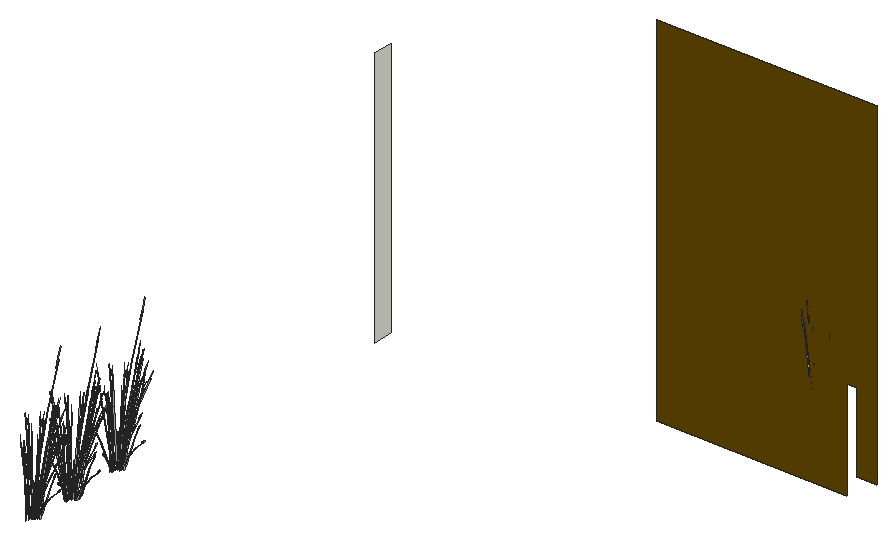
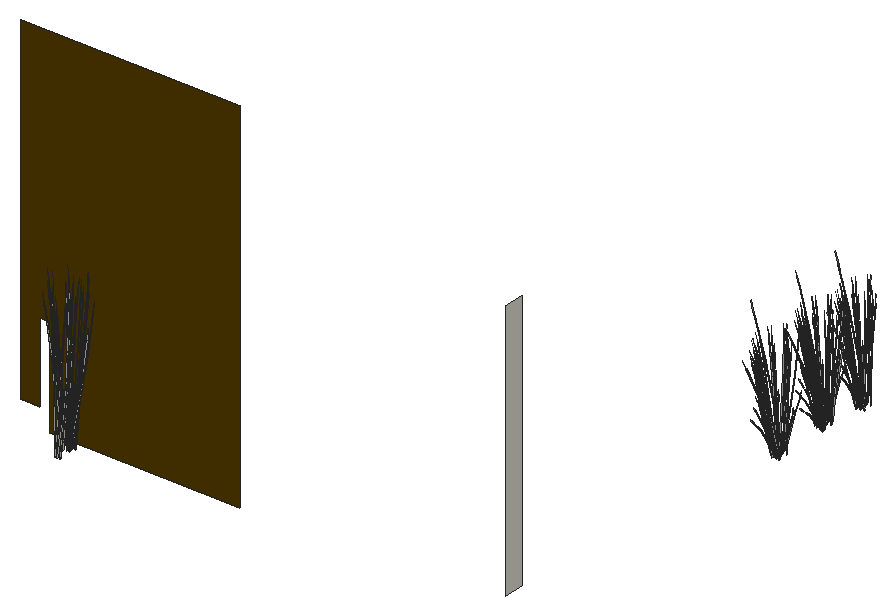
# SketchUp Ruby script. Lengths in inches.
U = 1.inch
M = Sketchup.active_model
def pt(a) = Geom::Point3d.new(a.map { |v| v * U })
def face(e, loops, mat)
  f = e.add_face(loops[0].map { |a| pt(a) })
  loops[1..].each { |l| e.add_face(l.map { |a| pt(a) }).erase! }
  f.material = f.back_material = mat if mat
  f
end
# faces: each face lists its corners as indices into pts; further lists are holes
def faces(e, pts, list, mat = nil) = list.each { |f| face(e, (f[0].is_a?(Array) ? f : [f]).map { |l| l.map { |i| pts[i] } }, mat) }
# xy, xz, yz: faces in a plane at the given z, y or x. An outline is a flat list of corners, or four numbers for a rectangle; further outlines are holes
def ring(l) = l.size == 4 ? [[l[0], l[1]], [l[2], l[1]], [l[2], l[3]], [l[0], l[3]]] : l.each_slice(2).to_a
def flat(e, list, mat, &to3) = list.each { |f| face(e, (f[0].is_a?(Array) ? f : [f]).map { |l| ring(l).map { |u, v| to3.(u, v) } }, mat) }
def xy(e, z, list, mat = nil) = flat(e, list, mat) { |x, y| [x, y, z] }
def xz(e, y, list, mat = nil) = flat(e, list, mat) { |x, z| [x, y, z] }
def yz(e, x, list, mat = nil) = flat(e, list, mat) { |y, z| [x, y, z] }
def lines(e, pts, list) = list.each { |a, b| e.add_line(pt(pts[a]), pt(pts[b])) }
# prism: a flat outline (further loops are holes) pulled along v
def prism(e, loops, v, mat = nil)
  f = face(e, loops, mat); d = Geom::Vector3d.new(v.map { |x| x * U })
  f.pushpull(f.normal.samedirection?(d) ? d.length : -d.length)
end
def box(e, o, s, mat = nil) = prism(e, [[o, [o[0] + s[0], o[1], o[2]], [o[0] + s[0], o[1] + s[1], o[2]], [o[0], o[1] + s[1], o[2]]]], [0, 0, s[2]], mat)
def at(x, y, z, deg = 0) = Geom::Transformation.translation(pt([x, y, z])) * Geom::Transformation.rotation(ORIGIN, Z_AXIS, deg.degrees)
def axes(o, x, y, z) = Geom::Transformation.new([*x, 0, *y, 0, *z, 0, *pt(o).to_a, 1])
def part(name) = M.definitions.add(name)
# library, detail: a bought-in or finely detailed component or shape, given as its bounding box
def library(name, o, s) = part(name).tap { |d| box(d.entities, o, s) }
def detail(e, o, s) = box(e.add_group.entities, o, s)
def put(e, d, t, mat = nil) = e.add_instance(d, t).tap { |i| i.material = mat if mat }
def group(e, t, mat = nil) = e.add_group.tap { |g| g.transformation = t; g.material = mat if mat }.entities
root = M.entities
M.materials.add("D01_Frost_White").color = [238, 238, 227]
M.materials.add("D08_Bronzed_Mustard").color = [102, 74, 0]
M.materials.add("LightPink_Translucent").color = [144, 107, 117]
M.materials["LightPink_Translucent"].alpha = 0.75
c1 = part("blade")
p = [[2.15,0.21,22],[0,0.17,0],[0.09,0.45,0],[2.18,0.31,22],[2.29,0.31,22],[0.38,0.45,0],
  [2.48,0.24,33],[2.49,0.24,33],[2.48,0.22,33]]
faces(c1.entities,p,[[0,1,2,3],[4,5,2,3],[6,3,4,7],[8,0,3,6]])
c2 = part("seeds")
p = [[0.3,-0.1,1.38],[-0.01,-0.03,1.59],[-0.01,-0.03,0.03],[0.14,-0.07,-0.07],[0.29,-0.03,3],[0.15,0.01,3.11]]
faces(c2.entities,p,[[0,1,2,3],[1,0,4,5]],"LightPink_Translucent")
c3 = part("blade with seeds")
put(c3.entities,c1,at(0,0,0))
put(c3.entities,c2,axes([2.4,0.25,30.99],[1.5799,-0.05474,1.17369],[-0.12525,1.92788,0.29478],[-0.07173,-0.02425,1.56792]))
xz(root,373,[[382,150,382,258,448,258,448,156,442,156,442,180,439,180,439,150]],"D08_Bronzed_Mustard")
yz(root,307,[[361,150,367,228]],"D01_Frost_White")
put(root,c3,axes([297.88,255.65,151],[0.30197,-0.1603,0.05432],[0.1478,0.29231,0.42765],[-0.02916,-0.12885,0.65209]))
put(root,c3,axes([296.1,245.72,150.27],[-0.09368,-0.15143,1.44779],[0.43286,-0.12749,0.11706],[0.09783,0.23774,0.61892]))
put(root,c3,axes([296.9,260.5,150.98],[0.05195,0.07595,1.47793],[0.41921,0.02984,-0.23373],[0.04216,0.1675,0.11853]))
put(root,c3,axes([296.28,277.23,151.25],[0.40102,-0.2196,-0.10273],[0.19707,0.38974,-0.57019],[0.05291,0.16424,0.8664]))
put(root,c3,axes([297.78,255.68,151],[0.4038,0.12331,0.40553],[-0.13808,0.40538,0.33437],[-0.02427,-0.15942,0.83914]))
put(root,c3,axes([298.33,272.88,150.98],[-0.04162,0.03603,1.49853],[-0.40776,-0.12155,-0.1416],[-0.01476,-0.15722,0.26519]))
put(root,c3,axes([298.01,273.92,151.25],[-0.45039,-0.02337,-0.10273],[0.01231,-0.44247,-0.57019],[0.03129,-0.17041,0.8664]))
put(root,c3,axes([297.12,259.47,151.27],[0.12355,-0.36271,0.29918],[0.36044,0.10579,-0.38624],[0.03305,0.14603,0.73904]))
put(root,c3,axes([296.51,246.37,151.27],[-0.06329,-0.37991,0.29918],[0.36182,-0.10032,-0.38624],[0.09718,0.10887,0.73904]))
put(root,c3,axes([296.75,244.18,150.78],[-0.35411,-0.24507,1.16821],[0.37391,-0.38156,0.50405],[0.11425,0.22994,1.12919]))
put(root,c3,axes([297.22,242.98,150.82],[0.27728,-0.24833,-0.29918],[0.26248,0.28355,0.38624],[0.03994,-0.14407,0.73904]))
put(root,c3,axes([296.16,246.9,150.98],[0.00121,-0.0571,1.49853],[0.35119,-0.25193,-0.1416],[0.12199,0.08992,0.26519]))
put(root,c3,axes([297.33,243.11,151],[0.33677,0.02198,0.05432],[-0.00923,0.33185,0.42765],[0.03524,-0.12712,0.65209]))
put(root,c3,axes([297.4,277.28,151],[-0.4076,0.10824,0.40553],[-0.07074,-0.4246,0.33437],[0.09586,0.12514,0.83914]))
put(root,c3,axes([297.22,243.08,151],[0.29182,0.32181,0.40553],[-0.3099,0.27755,0.33437],[0.05383,-0.15098,0.83914]))
put(root,c3,axes([297.32,277.37,151],[-0.18625,0.29962,0.05432],[-0.26523,-0.17444,0.42765],[0.08575,0.09606,0.65209]))
put(root,c3,axes([297,259.63,151.25],[0.40102,-0.2196,-0.10273],[0.19707,0.38974,-0.57019],[0.05291,0.16424,0.8664]))
put(root,c3,axes([296.85,276.38,150.27],[-0.09368,-0.15143,1.44779],[0.43286,-0.12749,0.11706],[0.09783,0.23774,0.61892]))
put(root,c3,axes([299.04,255.28,150.98],[-0.04162,0.03603,1.49853],[-0.40776,-0.12155,-0.1416],[-0.01476,-0.15722,0.26519]))
put(root,c3,axes([298.72,256.32,151.25],[-0.45039,-0.02337,-0.10273],[0.01231,-0.44247,-0.57019],[0.03129,-0.17041,0.8664]))
put(root,c3,axes([298.55,256.38,151.27],[-0.27728,0.24833,0.29918],[-0.26248,-0.28355,-0.38624],[0.03994,-0.14407,0.73904]))
put(root,c3,axes([297.56,244.1,151.27],[-0.35672,0.06741,0.29918],[-0.09419,-0.38534,-0.38624],[0.10222,-0.1035,0.73904]))
put(root,c3,axes([296.53,243.03,150.27],[-0.0763,0.16212,1.44779],[-0.3201,-0.3355,0.11706],[0.1444,-0.2091,0.61892]))
put(root,c3,axes([296.48,246.5625,151.25],[0.2442,-0.40372,-0.10273],[0.35364,0.23259,-0.57019],[0.12293,0.11406,0.8664]))
put(root,c3,axes([297.51,274.84,150.78],[-0.35411,-0.24507,1.16821],[0.37391,-0.38156,0.50405],[0.11425,0.22994,1.12919]))
put(root,c3,axes([297.98,273.64,150.82],[0.27728,-0.24833,-0.29918],[0.26248,0.28355,0.38624],[0.03994,-0.14407,0.73904]))
put(root,c3,axes([297.74,244.14,151.25],[-0.37908,-0.26007,-0.10273],[0.21839,-0.37663,-0.57019],[0.1071,-0.13092,0.8664]))
put(root,c3,axes([296.91,277.55,150.98],[0.00121,-0.0571,1.49853],[0.35119,-0.25193,-0.1416],[0.12199,0.08992,0.26519]))
put(root,c3,axes([298.08,273.77,151],[0.33677,0.02198,0.05432],[-0.00923,0.33185,0.42765],[0.03524,-0.12712,0.65209]))
put(root,c3,axes([298.12,259.68,151],[-0.4076,0.10824,0.40553],[-0.07074,-0.4246,0.33437],[0.09586,0.12514,0.83914]))
put(root,c3,axes([298.04,259.76,151],[-0.18625,0.29962,0.05432],[-0.26523,-0.17444,0.42765],[0.08575,0.09606,0.65209]))
put(root,c3,axes([298.42,273.22,150.98],[-0.00396,-0.09387,1.47793],[-0.33411,-0.2713,-0.23373],[0.05166,-0.16446,0.11853]))
put(root,c3,axes([297.57,258.77,150.27],[-0.09368,-0.15143,1.44779],[0.43286,-0.12749,0.11706],[0.09783,0.23774,0.61892]))
put(root,c3,axes([297.98,273.74,151],[0.29182,0.32181,0.40553],[-0.3099,0.27755,0.33437],[0.05383,-0.15098,0.83914]))
put(root,c3,axes([297.23,245.85,151.27],[-0.23317,-0.29531,0.29918],[0.26625,-0.27955,-0.38624],[0.13527,0.04253,0.73904]))
put(root,c3,axes([297.44,246.12,151],[-0.02064,0.35866,0.05432],[-0.3116,-0.00983,0.42765],[0.11936,0.03753,0.65209]))
put(root,c3,axes([297.47,246.01,151],[-0.30217,0.31079,0.40553],[-0.2606,-0.33005,0.33437],[0.14177,0.05733,0.83914]))
put(root,c3,axes([298.25,246.05,150.32],[-0.07843,-0.39649,-0.0295],[0.37072,-0.09115,-0.13375],[0.07742,0.02514,0.44114]))
put(root,c3,axes([297.61,245.03,151.27],[-0.34057,-0.13158,0.29918],[0.09933,-0.38387,-0.38624],[0.13712,-0.0352,0.73904]))
put(root,c3,axes([297.98,259.41,151.27],[-0.06329,-0.37991,0.29918],[0.36182,-0.10032,-0.38624],[0.09718,0.10887,0.73904]))
put(root,c3,axes([297.29,273.68,150.27],[-0.0763,0.16212,1.44779],[-0.3201,-0.3355,0.11706],[0.1444,-0.2091,0.61892]))
put(root,c3,axes([298.23,257.23,150.78],[-0.35411,-0.24507,1.16821],[0.37391,-0.38156,0.50405],[0.11425,0.22994,1.12919]))
put(root,c3,axes([297.88,244.04,151],[0.28133,0.19836,0.05432],[-0.16379,0.28248,0.42765],[0.0902,-0.09132,0.65209]))
put(root,c3,axes([297.23,277.22,151.25],[0.2442,-0.40372,-0.10273],[0.35364,0.23259,-0.57019],[0.12293,0.11406,0.8664]))
put(root,c3,axes([297.63,259.95,150.98],[0.00121,-0.0571,1.49853],[0.35119,-0.25193,-0.1416],[0.12199,0.08992,0.26519]))
put(root,c3,axes([298.8,256.16,151],[0.33677,0.02198,0.05432],[-0.00923,0.33185,0.42765],[0.03524,-0.12712,0.65209]))
put(root,c3,axes([298.5,274.79,151.25],[-0.37908,-0.26007,-0.10273],[0.21839,-0.37663,-0.57019],[0.1071,-0.13092,0.8664]))
put(root,c3,axes([297.8,243.96,151],[0.10163,0.43409,0.40553],[-0.39868,0.07534,0.33437],[0.1175,-0.10209,0.83914]))
put(root,c3,axes([299.13,255.61,150.98],[-0.00396,-0.09387,1.47793],[-0.33411,-0.2713,-0.23373],[0.05166,-0.16446,0.11853]))
put(root,c3,axes([298.69,256.13,151],[0.29182,0.32181,0.40553],[-0.3099,0.27755,0.33437],[0.05383,-0.15098,0.83914]))
put(root,c3,axes([296.72,245.25,150.27],[-0.15222,-0.08126,1.44779],[0.31502,-0.34091,0.11706],[0.19634,0.15379,0.61892]))
put(root,c3,axes([298.67,244.03,150.98],[-0.05353,-0.00358,1.49853],[-0.22227,-0.38383,-0.1416],[0.08926,-0.1262,0.26519]))
put(root,c3,axes([297.85,243.875,150.82],[0.35672,-0.06741,-0.29918],[0.09419,0.38534,0.38624],[0.10222,-0.1035,0.73904]))
put(root,c3,axes([298.2,276.78,151],[-0.02064,0.35866,0.05432],[-0.3116,-0.00983,0.42765],[0.11936,0.03753,0.65209]))
put(root,c3,axes([297.92,245.14,151],[0.15051,0.3216,0.05432],[-0.27447,0.15741,0.42765],[0.12099,-0.03106,0.65209]))
put(root,c3,axes([298.23,276.66,151],[-0.30217,0.31079,0.40553],[-0.2606,-0.33005,0.33437],[0.14177,0.05733,0.83914]))
put(root,c3,axes([297.29,246.04,151.25],[0.02194,-0.47967,-0.10273],[0.41546,0.01311,-0.57019],[0.16001,0.03332,0.8664]))
put(root,c3,axes([297.76,245.15,151.25],[-0.20619,-0.42709,-0.10273],[0.36595,-0.20988,-0.57019],[0.15422,-0.05635,0.8664]))
put(root,c3,axes([299.03,257.15,151.27],[-0.35672,0.06741,0.29918],[-0.09419,-0.38534,-0.38624],[0.10222,-0.1035,0.73904]))
put(root,c3,axes([297.89,245.03,151],[-0.11578,0.43006,0.40553],[-0.38064,-0.14706,0.33437],[0.14969,-0.02584,0.83914]))
put(root,c3,axes([299.01,276.71,150.32],[-0.07843,-0.39649,-0.0295],[0.37072,-0.09115,-0.13375],[0.07742,0.02514,0.44114]))
put(root,c3,axes([298,256.07,150.27],[-0.0763,0.16212,1.44779],[-0.3201,-0.3355,0.11706],[0.1444,-0.2091,0.61892]))
put(root,c3,axes([297.95,259.61,151.25],[0.2442,-0.40372,-0.10273],[0.35364,0.23259,-0.57019],[0.12293,0.11406,0.8664]))
put(root,c3,axes([298.64,274.7,151],[0.28133,0.19836,0.05432],[-0.16379,0.28248,0.42765],[0.0902,-0.09132,0.65209]))
put(root,c3,axes([299.21,257.1875,151.25],[-0.37908,-0.26007,-0.10273],[0.21839,-0.37663,-0.57019],[0.1071,-0.13092,0.8664]))
put(root,c3,axes([297.65,245.75,150.98],[0.08791,-0.00798,1.47793],[0.24113,-0.36643,-0.23373],[0.15637,0.04837,0.11853]))
put(root,c3,axes([298.56,274.61,151],[0.10163,0.43409,0.40553],[-0.39868,0.07534,0.33437],[0.1175,-0.10209,0.83914]))
put(root,c3,axes([298.7,258.9,151.27],[-0.23317,-0.29531,0.29918],[0.26625,-0.27955,-0.38624],[0.13527,0.04253,0.73904]))
put(root,c3,axes([297.48,275.91,150.27],[-0.15222,-0.08126,1.44779],[0.31502,-0.34091,0.11706],[0.19634,0.15379,0.61892]))
put(root,c3,axes([297.97,244.98,150.82],[0.34057,0.13158,-0.29918],[-0.09933,0.38387,0.38624],[0.13712,-0.0352,0.73904]))
put(root,c3,axes([299.43,274.68,150.98],[-0.05353,-0.00358,1.49853],[-0.22227,-0.38383,-0.1416],[0.08926,-0.1262,0.26519]))
put(root,c3,axes([298.91,259.17,151],[-0.02064,0.35866,0.05432],[-0.3116,-0.00983,0.42765],[0.11936,0.03753,0.65209]))
put(root,c3,axes([298.61,274.53,150.82],[0.35672,-0.06741,-0.29918],[0.09419,0.38534,0.38624],[0.10222,-0.1035,0.73904]))
put(root,c3,axes([298.94,259.06,151],[-0.30217,0.31079,0.40553],[-0.2606,-0.33005,0.33437],[0.14177,0.05733,0.83914]))
put(root,c3,axes([298.68,275.8,151],[0.15051,0.3216,0.05432],[-0.27447,0.15741,0.42765],[0.12099,-0.03106,0.65209]))
put(root,c3,axes([298.32,276.66,150.82],[0.23317,0.29531,-0.29918],[-0.26625,0.27955,0.38624],[0.13527,0.04253,0.73904]))
put(root,c3,axes([298.05,276.7,151.25],[0.02194,-0.47967,-0.10273],[0.41546,0.01311,-0.57019],[0.16001,0.03332,0.8664]))
put(root,c3,axes([298.51,275.81,151.25],[-0.20619,-0.42709,-0.10273],[0.36595,-0.20988,-0.57019],[0.15422,-0.05635,0.8664]))
put(root,c3,axes([299.73,259.1,150.32],[-0.07843,-0.39649,-0.0295],[0.37072,-0.09115,-0.13375],[0.07742,0.02514,0.44114]))
put(root,c3,axes([299.09,258.07,151.27],[-0.34057,-0.13158,0.29918],[0.09933,-0.38387,-0.38624],[0.13712,-0.0352,0.73904]))
put(root,c3,axes([298.65,275.68,151],[-0.11578,0.43006,0.40553],[-0.38064,-0.14706,0.33437],[0.14969,-0.02584,0.83914]))
put(root,c3,axes([298.58,246.42,150.98],[-0.03706,-0.04129,1.49853],[0.08106,-0.44261,-0.1416],[0.14596,-0.02828,0.26519]))
put(root,c3,axes([297.04,244.51,150.27],[-0.16998,0.01068,1.44779],[0.11276,-0.46299,0.11706],[0.24224,0.02864,0.61892]))
put(root,c3,axes([299.35,257.09,151],[0.28133,0.19836,0.05432],[-0.16379,0.28248,0.42765],[0.0902,-0.09132,0.65209]))
put(root,c3,axes([298.41,276.41,150.98],[0.08791,-0.00798,1.47793],[0.24113,-0.36643,-0.23373],[0.15637,0.04837,0.11853]))
put(root,c3,axes([299.27,257.01,151],[0.10163,0.43409,0.40553],[-0.39868,0.07534,0.33437],[0.1175,-0.10209,0.83914]))
put(root,c3,axes([298.875,244.48,150.98],[0.05687,-0.07184,1.47793],[-0.07279,-0.44069,-0.23373],[0.14268,-0.08356,0.11853]))
put(root,c3,axes([298.2,258.3,150.27],[-0.15222,-0.08126,1.44779],[0.31502,-0.34091,0.11706],[0.19634,0.15379,0.61892]))
put(root,c3,axes([300.15,257.07,150.98],[-0.05353,-0.00358,1.49853],[-0.22227,-0.38383,-0.1416],[0.08926,-0.1262,0.26519]))
put(root,c3,axes([298.73,275.64,150.82],[0.34057,0.13158,-0.29918],[-0.09933,0.38387,0.38624],[0.13712,-0.0352,0.73904]))
put(root,c3,axes([299.4,258.19,151],[0.15051,0.3216,0.05432],[-0.27447,0.15741,0.42765],[0.12099,-0.03106,0.65209]))
put(root,c3,axes([298.77,259.09,151.25],[0.02194,-0.47967,-0.10273],[0.41546,0.01311,-0.57019],[0.16001,0.03332,0.8664]))
put(root,c3,axes([299.23,258.2,151.25],[-0.20619,-0.42709,-0.10273],[0.36595,-0.20988,-0.57019],[0.15422,-0.05635,0.8664]))
put(root,c3,axes([299.37,258.08,151],[-0.11578,0.43006,0.40553],[-0.38064,-0.14706,0.33437],[0.14969,-0.02584,0.83914]))
put(root,c3,axes([299.33,277.08,150.98],[-0.03706,-0.04129,1.49853],[0.08106,-0.44261,-0.1416],[0.14596,-0.02828,0.26519]))
put(root,c3,axes([297.8,275.16,150.27],[-0.16998,0.01068,1.44779],[0.11276,-0.46299,0.11706],[0.24224,0.02864,0.61892]))
put(root,c3,axes([299.13,258.8,150.98],[0.08791,-0.00798,1.47793],[0.24113,-0.36643,-0.23373],[0.15637,0.04837,0.11853]))
put(root,c3,axes([299.63,275.14,150.98],[0.05687,-0.07184,1.47793],[-0.07279,-0.44069,-0.23373],[0.14268,-0.08356,0.11853]))
put(root,c3,axes([300.05,259.47,150.98],[-0.03706,-0.04129,1.49853],[0.08106,-0.44261,-0.1416],[0.14596,-0.02828,0.26519]))
put(root,c3,axes([298.52,257.56,150.27],[-0.16998,0.01068,1.44779],[0.11276,-0.46299,0.11706],[0.24224,0.02864,0.61892]))
put(root,c3,axes([300.35,257.53,150.98],[0.05687,-0.07184,1.47793],[-0.07279,-0.44069,-0.23373],[0.14268,-0.08356,0.11853]))
put(root,c3,axes([428.51,378.72,151.74],[-0.42629,-0.07733,-0.52676],[0.08996,-0.47699,-0.13825],[-0.12722,-0.0578,1.16273]))
put(root,c3,axes([427.96,379.62,151.7],[-0.38354,-0.23583,-0.41945],[0.22925,-0.42288,0],[-0.08735,-0.05371,1.33059]))
put(root,c3,axes([428.0625,379.44,151.71],[-0.09626,-0.41098,-0.2617],[0.38233,-0.1167,0.2617],[-0.07708,-0.04739,1.17405]))
put(root,c3,axes([429.27,379.13,151.74],[-0.27603,0.35451,-0.52676],[-0.34289,-0.32147,-0.13825],[-0.11061,0.08844,1.16273]))
put(root,c3,axes([428.74,378.57,151.87],[-0.24618,-0.39589,-0.37796],[0.37289,-0.27878,0.1819],[-0.07967,-0.04899,1.2135]))
put(root,c3,axes([429.26,378.85,151.87],[-0.44501,0.02912,-0.37796],[-0.04024,-0.48332,0.1819],[-0.07967,0.04899,1.2135]))
put(root,c3,axes([429.73,380.1,151.7],[-0.38354,0.23583,-0.41945],[-0.22925,-0.42288,0],[-0.08735,0.05371,1.33059]))
put(root,c3,axes([427.46,377.75,151.7],[0,-0.47166,-0.41945],[0.45849,0,0],[0,-0.10742,1.33059]))
put(root,c3,axes([427.46,383.5,151.7],[0,-0.47166,-0.41945],[0.45849,0,0],[0,-0.10742,1.33059]))
put(root,c3,axes([429.64,379.91,151.71],[-0.38233,-0.1167,-0.2617],[0.09626,-0.41098,0.2617],[-0.07708,0.04739,1.17405]))
put(root,c3,axes([428.45,377.82,151.77],[-0.1683,-0.48366,-0.58997],[0.48479,-0.17419,-0.15484],[-0.0186,-0.16378,1.30225]))
put(root,c3,axes([428.45,383.5625,151.77],[-0.1683,-0.48366,-0.58997],[0.48479,-0.17419,-0.15484],[-0.0186,-0.16378,1.30225]))
put(root,c3,axes([427.65,377.76,151.71],[0.28606,-0.29428,-0.2617],[0.28606,0.29428,0.2617],[0,-0.09479,1.17405]))
put(root,c3,axes([428.7,377.94,151.87],[0.19883,-0.425,-0.37796],[0.41314,0.20454,0.1819],[0,-0.09797,1.2135]))
put(root,c3,axes([428.7,383.6875,151.87],[0.19883,-0.425,-0.37796],[0.41314,0.20454,0.1819],[0,-0.09797,1.2135]))
put(root,c3,axes([429.75,378.51,151.87],[-0.19883,0.425,-0.37796],[-0.41314,-0.20454,0.1819],[0,0.09797,1.2135]))
put(root,c3,axes([430.8,378.69,151.71],[-0.28606,0.29428,-0.2617],[-0.28606,-0.29428,0.2617],[0,0.09479,1.17405]))
put(root,c3,axes([428.82,376.54,151.71],[0.38233,0.1167,-0.2617],[-0.09626,0.41098,0.2617],[0.07708,-0.04739,1.17405]))
put(root,c3,axes([431,378.7,151.7],[0,0.47166,-0.41945],[-0.45849,0,0],[0,0.10742,1.33059]))
put(root,c3,axes([428.73,376.35,151.7],[0.38354,-0.23583,-0.41945],[0.22925,0.42288,0],[0.08735,-0.05371,1.33059]))
put(root,c3,axes([428.73,382.1,151.7],[0.38354,-0.23583,-0.41945],[0.22925,0.42288,0],[0.08735,-0.05371,1.33059]))
put(root,c3,axes([429.72,377.88,151.87],[0.24618,0.39589,-0.37796],[-0.37289,0.27878,0.1819],[0.07967,0.04899,1.2135]))
put(root,c3,axes([429.19,377.32,151.74],[0.27603,-0.35451,-0.52676],[0.34289,0.32147,-0.13825],[0.11061,-0.08844,1.16273]))
put(root,c3,axes([429.19,383.07,151.74],[0.27603,-0.35451,-0.52676],[0.34289,0.32147,-0.13825],[0.11061,-0.08844,1.16273]))
put(root,c3,axes([430.4,377,151.71],[0.09626,0.41098,-0.2617],[-0.38233,0.1167,0.2617],[0.07708,0.04739,1.17405]))
put(root,c3,axes([430.5,376.83,151.7],[0.38354,0.23583,-0.41945],[-0.22925,0.42288,0],[0.08735,0.05371,1.33059]))
put(root,c3,axes([429.94,377.73,151.74],[0.42629,0.07733,-0.52676],[-0.08996,0.47699,-0.13825],[0.12722,0.0578,1.16273]))
